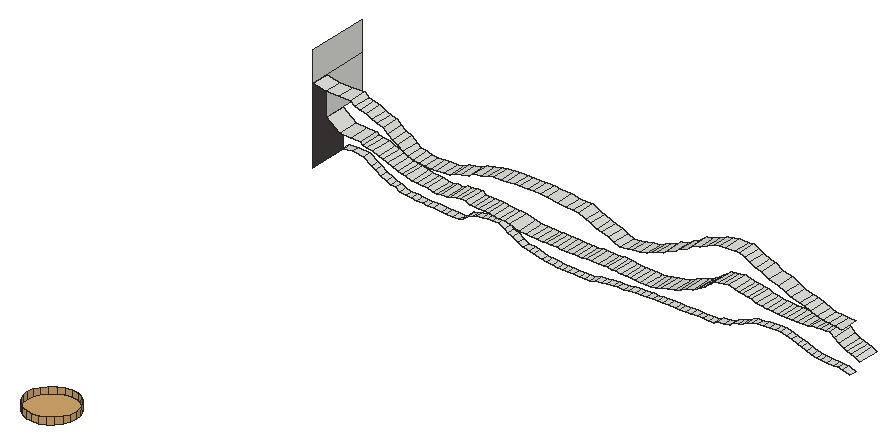
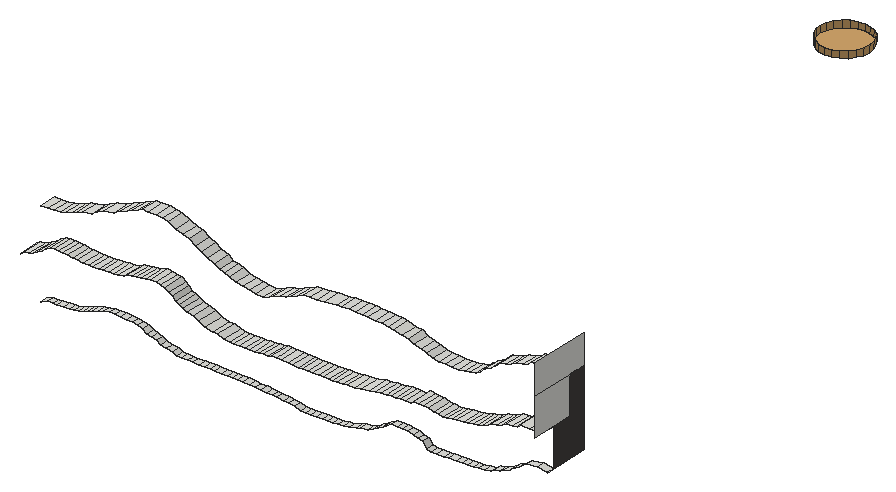
# SketchUp Ruby script. Lengths in inches.
U = 1.inch
M = Sketchup.active_model
def pt(a) = Geom::Point3d.new(a.map { |v| v * U })
def face(e, loops, mat)
  f = e.add_face(loops[0].map { |a| pt(a) })
  loops[1..].each { |l| e.add_face(l.map { |a| pt(a) }).erase! }
  f.material = f.back_material = mat if mat
  f
end
# faces: each face lists its corners as indices into pts; further lists are holes
def faces(e, pts, list, mat = nil) = list.each { |f| face(e, (f[0].is_a?(Array) ? f : [f]).map { |l| l.map { |i| pts[i] } }, mat) }
# xy, xz, yz: faces in a plane at the given z, y or x. An outline is a flat list of corners, or four numbers for a rectangle; further outlines are holes
def ring(l) = l.size == 4 ? [[l[0], l[1]], [l[2], l[1]], [l[2], l[3]], [l[0], l[3]]] : l.each_slice(2).to_a
def flat(e, list, mat, &to3) = list.each { |f| face(e, (f[0].is_a?(Array) ? f : [f]).map { |l| ring(l).map { |u, v| to3.(u, v) } }, mat) }
def xy(e, z, list, mat = nil) = flat(e, list, mat) { |x, y| [x, y, z] }
def xz(e, y, list, mat = nil) = flat(e, list, mat) { |x, z| [x, y, z] }
def yz(e, x, list, mat = nil) = flat(e, list, mat) { |y, z| [x, y, z] }
def lines(e, pts, list) = list.each { |a, b| e.add_line(pt(pts[a]), pt(pts[b])) }
# prism: a flat outline (further loops are holes) pulled along v
def prism(e, loops, v, mat = nil)
  f = face(e, loops, mat); d = Geom::Vector3d.new(v.map { |x| x * U })
  f.pushpull(f.normal.samedirection?(d) ? d.length : -d.length)
end
def box(e, o, s, mat = nil) = prism(e, [[o, [o[0] + s[0], o[1], o[2]], [o[0] + s[0], o[1] + s[1], o[2]], [o[0], o[1] + s[1], o[2]]]], [0, 0, s[2]], mat)
def at(x, y, z, deg = 0) = Geom::Transformation.translation(pt([x, y, z])) * Geom::Transformation.rotation(ORIGIN, Z_AXIS, deg.degrees)
def axes(o, x, y, z) = Geom::Transformation.new([*x, 0, *y, 0, *z, 0, *pt(o).to_a, 1])
def part(name) = M.definitions.add(name)
# library, detail: a bought-in or finely detailed component or shape, given as its bounding box
def library(name, o, s) = part(name).tap { |d| box(d.entities, o, s) }
def detail(e, o, s) = box(e.add_group.entities, o, s)
def put(e, d, t, mat = nil) = e.add_instance(d, t).tap { |i| i.material = mat if mat }
def group(e, t, mat = nil) = e.add_group.tap { |g| g.transformation = t; g.material = mat if mat }.entities
root = M.entities
M.materials.add("[Field Square Tile]").color = [211, 167, 108]
M.materials.add("[Granite Tile]1").color = [68, 65, 63]
xy(root,237.65,[[2039.58,565.74,2040.27,566.68],[2040.27,565.74,2040.89,566.68]])
xy(root,238.33,[[2048.68,565.74,2049.23,566.68],[2049.23,565.74,2049.91,566.68]])
xy(root,238.34,[[2050.59,565.74,2051.52,566.68],[2051.52,565.74,2052.01,566.68],[2052.01,565.74,2052.77,566.68],[2052.77,565.74,2053.4,566.68],[2053.4,565.74,2054.15,566.68],
  [2054.15,565.74,2054.77,566.68],[2054.77,565.74,2055.54,566.68],[2055.54,565.74,2056.16,566.68]])
xy(root,241.52,[[2010.28,561.05,2010.34,566.68]])
xy(root,241.68,[[2040.78,563.18,2041.37,565.74]])
xy(root,241.75,[[2043.13,563.18,2044,565.74],[2044,563.18,2044.62,565.74],[2044.62,563.18,2045.13,565.74]])
xy(root,250.6875,[[2030.6,492.27,2029.81,492.375,2029.07,492.68,2028.43,493.17,2027.95,493.8,2027.64,494.54,2027.54,495.33,2027.64,496.125,2027.95,496.86,2028.43,497.5,2029.07,497.98,2029.81,498.29,2030.6,498.39,2031.39,498.29,2032.13,497.98,2032.76,497.5,2033.25,496.86,2033.56,496.125,2033.66,495.33,2033.56,494.54,2033.25,493.8,2032.76,493.17,2032.13,492.68,2031.39,492.375]],"[Field Square Tile]")
xz(root,561.05,[[2010.28,241.52,2010.34,251.5]])
yz(root,2010.34,[[563.18,246.2,568.68,250.88],[561.05,250.88,568.68,254.5]])
yz(root,2010.34,[[561.05,241.52,565.74,241.52,565.74,246.2,563.18,246.2,563.18,250.88,561.05,250.88]],"[Granite Tile]1")
p = [[2040.89,565.74,237.65],[2040.89,566.68,237.65],[2041.56,566.68,237.89],[2041.56,565.74,237.89],[2036.22,565.74,237.76],[2036.22,566.68,237.76],
  [2036.93,566.68,237.71],[2036.93,565.74,237.71],[2037.54,566.68,237.68],[2037.54,565.74,237.68],[2038.14,566.68,237.67],[2038.14,565.74,237.67],
  [2038.89,566.68,237.66],[2038.89,565.74,237.66],[2039.58,566.68,237.65],[2039.58,565.74,237.65],[2034.87,565.74,237.9],[2034.87,566.68,237.9],
  [2035.53,566.68,237.82],[2035.53,565.74,237.82],[2033.93,565.74,238.21],[2033.93,566.68,238.21],[2042.32,566.68,237.94],[2042.32,565.74,237.94],
  [2042.9375,566.68,237.98],[2042.9375,565.74,237.98],[2043.79,566.68,238.1],[2043.79,565.74,238.1],[2044.34,566.68,238.13],[2044.34,565.74,238.13],
  [2045.1,566.68,238.15],[2045.1,565.74,238.15],[2033.46,565.74,238.31],[2033.46,566.68,238.31],[2045.73,566.68,238.26],[2045.73,565.74,238.26],
  [2032.55,565.74,238.43],[2032.55,566.68,238.43],[2046.48,566.68,238.28],[2046.48,565.74,238.28],[2047.11,566.68,238.3],[2047.11,565.74,238.3],
  [2047.96,566.68,238.32],[2047.96,565.74,238.32],[2048.68,566.68,238.33],[2048.68,565.74,238.33],[2049.91,565.74,238.33],[2049.91,566.68,238.33],
  [2050.59,566.68,238.34],[2050.59,565.74,238.34],[2056.16,565.74,238.34],[2056.16,566.68,238.34],[2056.67,566.68,238.59],[2056.67,565.74,238.59],
  [2031.9,565.74,238.74],[2031.9,566.68,238.74],[2072.19,565.74,238.78],[2072.19,566.68,238.78],[2072.97,566.68,238.43],[2072.97,565.74,238.43],
  [2057.49,566.68,238.72],[2057.49,565.74,238.72],[2031.32,565.74,239.11],[2031.32,566.68,239.11],[2058.18,566.68,238.86],[2058.18,565.74,238.86],
  [2021.53,565.74,238.92],[2021.53,566.68,238.92],[2022.57,566.68,238.82],[2022.57,565.74,238.82],[2023.08,566.68,238.8],[2023.08,565.74,238.8],
  [2023.95,566.68,238.79],[2023.95,565.74,238.79],[2024.69,566.68,238.77],[2024.69,565.74,238.77],[2025.22,566.68,238.9375],[2025.22,565.74,238.9375],
  [2069.47,565.74,238.875],[2069.47,566.68,238.875],[2070.22,566.68,238.83],[2070.22,565.74,238.83],[2070.98,566.68,238.8],[2070.98,565.74,238.8],
  [2071.52,566.68,238.79],[2071.52,565.74,238.79],[2019.44,565.74,238.97],[2019.44,566.68,238.97],[2020.14,566.68,238.94],[2020.14,565.74,238.94],
  [2020.84,566.68,238.93],[2020.84,565.74,238.93],[2025.78,566.68,239.55],[2025.78,565.74,239.55],[2058.69,566.68,239.18],[2058.69,565.74,239.18],
  [2068.32,565.74,239.04],[2068.32,566.68,239.04],[2068.9,566.68,238.94],[2068.9,565.74,238.94],[2018.07,565.74,239.09],[2018.07,566.68,239.09],
  [2018.76,566.68,239.03],[2018.76,565.74,239.03],[2067.66,565.74,239.29],[2067.66,566.68,239.29],[2017.29,565.74,239.19],[2017.29,566.68,239.19],
  [2030.74,565.74,239.38],[2030.74,566.68,239.38],[2016.78,565.74,239.52],[2016.78,566.68,239.52],[2059.28,566.68,239.35],[2059.28,565.74,239.35],
  [2067.08,565.74,239.53],[2067.08,566.68,239.53],[2030.28,565.74,239.71],[2030.28,566.68,239.71],[2059.84,566.68,239.52],[2059.84,565.74,239.52],
  [2016.22,565.74,239.64],[2016.22,566.68,239.64],[2060.39,566.68,239.85],[2060.39,565.74,239.85],[2066.55,565.74,239.7],[2066.55,566.68,239.7],
  [2015.77,565.74,239.86],[2015.77,566.68,239.86],[2026.36,566.68,239.69],[2026.36,565.74,239.69],[2026.91,566.68,239.88],[2026.91,565.74,239.88],
  [2029.58,565.74,240.11],[2029.58,566.68,240.11],[2065.86,565.74,239.92],[2065.86,566.68,239.92],[2061.03,566.68,240.03],[2061.03,565.74,240.03],
  [2014.98,565.74,240.2],[2014.98,566.68,240.2],[2027.64,566.68,239.99],[2027.64,565.74,239.99],[2065.23,565.74,240.11],[2065.23,566.68,240.11],
  [2028.23,566.68,240.05],[2028.23,565.74,240.05],[2028.89,566.68,240.09],[2028.89,565.74,240.09],[2061.6875,566.68,240.12],[2061.6875,565.74,240.12],
  [2062.36,566.68,240.19],[2062.36,565.74,240.19],[2064.45,565.74,240.27],[2064.45,566.68,240.27],[2014.38,565.74,240.59],[2014.38,566.68,240.59],
  [2063.125,566.68,240.23],[2063.125,565.74,240.23],[2063.83,566.68,240.25],[2063.83,565.74,240.25],[2013.84,565.74,240.85],[2013.84,566.68,240.85],
  [2012.82,565.74,241.55],[2012.82,566.68,241.55],[2046.76,563.18,241.57],[2046.76,565.74,241.57],[2047.3,565.74,241.53],[2047.3,563.18,241.53],
  [2047.92,565.74,241.51],[2047.92,563.18,241.51],[2048.47,565.74,241.49],[2048.47,563.18,241.49],[2049.17,565.74,241.48],[2049.17,563.18,241.48],
  [2049.83,565.74,241.47],[2049.83,563.18,241.47],[2050.4,565.74,241.46],[2050.4,563.18,241.46],[2051.11,565.74,241.6],[2051.11,563.18,241.6],
  [2010.34,565.74,241.52],[2010.34,566.68,241.52],[2011.55,566.68,241.69],[2011.55,565.74,241.69],[2046.15,563.18,241.66],[2046.15,565.74,241.66],
  [2051.84,565.74,241.85],[2051.84,563.18,241.85],[2037.12,563.18,241.75],[2037.12,565.74,241.75],[2037.57,565.74,241.74],[2037.57,563.18,241.74],
  [2038.12,565.74,241.72],[2038.12,563.18,241.72],[2038.75,565.74,241.71],[2038.75,563.18,241.71],[2039.38,565.74,241.7],[2039.38,563.18,241.7],
  [2040.11,565.74,241.69],[2040.11,563.18,241.69],[2040.78,565.74,241.68],[2040.78,563.18,241.68],[2041.37,563.18,241.68],[2041.37,565.74,241.68],
  [2041.86,565.74,241.67],[2041.86,563.18,241.67],[2042.5625,565.74,241.74],[2042.5625,563.18,241.74],[2043.13,565.74,241.75],[2043.13,563.18,241.75],
  [2045.13,563.18,241.75],[2045.13,565.74,241.75],[2045.62,565.74,241.67],[2045.62,563.18,241.67],[2034.93,563.18,241.89],[2034.93,565.74,241.89],
  [2035.75,565.74,241.83],[2035.75,563.18,241.83],[2036.35,565.74,241.78],[2036.35,563.18,241.78],[2052.51,565.74,241.91],[2052.51,563.18,241.91],
  [2034.16,563.18,241.96],[2034.16,565.74,241.96],[2053.41,565.74,242.1],[2053.41,563.18,242.1],[2032.99,563.18,242.24],[2032.99,565.74,242.24],
  [2054.18,565.74,242.46],[2054.18,563.18,242.46],[2032.32,563.18,242.34],[2032.32,565.74,242.34],[2075.79,563.18,242.51],[2075.79,565.74,242.51],
  [2076.3,565.74,242.21],[2076.3,563.18,242.21],[2031.66,563.18,242.38],[2031.66,565.74,242.38],[2031,563.18,242.48],[2031,565.74,242.48],
  [2022.82,563.18,242.68],[2022.82,565.74,242.68],[2023.49,565.74,242.51],[2023.49,563.18,242.51],[2024.01,565.74,242.46],[2024.01,563.18,242.46],
  [2024.55,565.74,242.58],[2024.55,563.18,242.58],[2030.36,563.18,242.57],[2030.36,565.74,242.57],[2054.88,565.74,242.78],[2054.88,563.18,242.78],
  [2075.2,563.18,242.68],[2075.2,565.74,242.68],[2025.18,565.74,242.57],[2025.18,563.18,242.57],[2025.81,565.74,242.81],[2025.81,563.18,242.81],
  [2027.58,563.18,242.92],[2027.58,565.74,242.92],[2028.01,565.74,242.625],[2028.01,563.18,242.625],[2028.62,565.74,242.65],[2028.62,563.18,242.65],
  [2029.17,565.74,242.62],[2029.17,563.18,242.62],[2029.8,565.74,242.58],[2029.8,563.18,242.58],[2021.47,563.18,242.78],[2021.47,565.74,242.78],
  [2022.28,565.74,242.73],[2022.28,563.18,242.73],[2074.7,563.18,242.875],[2074.7,565.74,242.875],[2020.17,563.18,243.06],[2020.17,565.74,243.06],
  [2020.89,565.74,242.85],[2020.89,563.18,242.85],[2026.38,565.74,242.86],[2026.38,563.18,242.86],[2055.65,565.74,242.97],[2055.65,563.18,242.97],
  [2026.94,565.74,242.89],[2026.94,563.18,242.89],[2074.31,563.18,243.09],[2074.31,565.74,243.09],[2056.18,565.74,243.23],[2056.18,563.18,243.23],
  [2019.1,563.18,243.3],[2019.1,565.74,243.3],[2019.6875,565.74,243.14],[2019.6875,563.18,243.14],[2073.7,563.18,243.43],[2073.7,565.74,243.43],
  [2056.58,565.74,243.48],[2056.58,563.18,243.48],[2018.46,563.18,243.48],[2018.46,565.74,243.48],[2073.16,563.18,243.8],[2073.16,565.74,243.8],
  [2017.94,563.18,243.79],[2017.94,565.74,243.79],[2057.1,565.74,243.72],[2057.1,563.18,243.72],[2057.4375,565.74,244.12],[2057.4375,563.18,244.12],
  [2017.28,563.18,243.95],[2017.28,565.74,243.95],[2072.56,563.18,244.18],[2072.56,565.74,244.18],[2016.76,563.18,244.11],[2016.76,565.74,244.11],
  [2065.38,563.18,243.99],[2065.38,565.74,243.99],[2066.1,565.74,243.95],[2066.1,563.18,243.95],[2066.6,565.74,243.93],[2066.6,563.18,243.93],
  [2067.29,565.74,243.91],[2067.29,563.18,243.91],[2067.86,565.74,243.89],[2067.86,563.18,243.89],[2068.56,565.74,243.88],[2068.56,563.18,243.88],
  [2069.21,565.74,243.94],[2069.21,563.18,243.94],[2069.85,565.74,243.95],[2069.85,563.18,243.95],[2070.41,565.74,244.1],[2070.41,563.18,244.1],
  [2064.2,563.18,244.11],[2064.2,565.74,244.11],[2064.76,565.74,244.04],[2064.76,563.18,244.04],[2016.09,563.18,244.41],[2016.09,565.74,244.41],
  [2057.91,565.74,244.39],[2057.91,563.18,244.39],[2063.45,563.18,244.25],[2063.45,565.74,244.25],[2071.04,565.74,244.13],[2071.04,563.18,244.13],
  [2071.52,565.74,244.15],[2071.52,563.18,244.15],[2072.04,565.74,244.17],[2072.04,563.18,244.17],[2062.99,563.18,244.51],[2062.99,565.74,244.51],
  [2015.33,563.18,244.54],[2015.33,565.74,244.54],[2058.39,565.74,244.73],[2058.39,563.18,244.73],[2014.77,563.18,244.61],[2014.77,565.74,244.61],
  [2061.84,563.18,244.67],[2061.84,565.74,244.67],[2062.45,565.74,244.55],[2062.45,563.18,244.55],[2014.55,563.18,244.92],[2014.55,565.74,244.92],
  [2058.875,565.74,244.87],[2058.875,563.18,244.87],[2060.79,563.18,244.81],[2060.79,565.74,244.81],[2061.36,565.74,244.7],[2061.36,563.18,244.7],
  [2060.14,563.18,245.01],[2060.14,565.74,245.01],[2011.91,563.18,244.96],[2011.91,565.74,244.96],[2013.3,565.74,244.9375],[2013.3,563.18,244.9375],
  [2059.46,565.74,244.95],[2059.46,563.18,244.95],[2010.34,563.18,246.2],[2010.34,565.74,246.2],[2047.59,561.05,246.35],[2047.59,563.18,246.35],
  [2048.36,563.18,246.05],[2048.36,561.05,246.05],[2049.26,563.18,246.13],[2049.26,561.05,246.13],[2049.97,563.18,246.29],[2049.97,561.05,246.29],
  [2050.77,563.18,246.41],[2050.77,561.05,246.41],[2046.98,561.05,246.66],[2046.98,563.18,246.66],[2051.68,563.18,246.55],[2051.68,561.05,246.55],
  [2023.4,561.05,246.62],[2023.4,563.18,246.62],[2024.14,563.18,246.54],[2024.14,561.05,246.54],[2024.92,563.18,246.51],[2024.92,561.05,246.51],
  [2025.7,563.18,246.58],[2025.7,561.05,246.58],[2074.89,561.05,246.59],[2074.89,563.18,246.59],[2075.78,563.18,246.55],[2075.78,561.05,246.55],
  [2022.74,561.05,246.73],[2022.74,563.18,246.73],[2026.5,563.18,246.59],[2026.5,561.05,246.59],[2027.3,563.18,246.69],[2027.3,561.05,246.69],
  [2052.41,563.18,246.92],[2052.41,561.05,246.92],[2074.18,561.05,246.66],[2074.18,563.18,246.66],[2022.02,561.05,246.88],[2022.02,563.18,246.88],
  [2028.01,563.18,247.03],[2028.01,561.05,247.03],[2046.125,561.05,246.94],[2046.125,563.18,246.94],[2073.39,561.05,246.75],[2073.39,563.18,246.75],
  [2072.7,561.05,246.95],[2072.7,563.18,246.95],[2021.47,561.05,247.25],[2021.47,563.18,247.25],[2045.44,561.05,247.08],[2045.44,563.18,247.08],
  [2053.02,563.18,247.12],[2053.02,561.05,247.12],[2028.7,563.18,247.2],[2028.7,561.05,247.2],[2071.89,561.05,247.25],[2071.89,563.18,247.25],
  [2044.76,561.05,247.46],[2044.76,563.18,247.46],[2053.7,563.18,247.31],[2053.7,561.05,247.31],[2029.67,563.18,247.39],[2029.67,561.05,247.39],
  [2071.21,561.05,247.53],[2071.21,563.18,247.53],[2020.83,561.05,247.72],[2020.83,563.18,247.72],[2054.27,563.18,247.71],[2054.27,561.05,247.71],
  [2030.3,563.18,247.78],[2030.3,561.05,247.78],[2044.13,561.05,247.66],[2044.13,563.18,247.66],[2070.63,561.05,247.66],[2070.63,563.18,247.66],
  [2020.18,561.05,248.07],[2020.18,563.18,248.07],[2043.29,561.05,248.08],[2043.29,563.18,248.08],[2055.2,563.18,248.03],[2055.2,561.05,248.03],
  [2069.5,561.05,247.9],[2069.5,563.18,247.9],[2031.08,563.18,247.89],[2031.08,561.05,247.89],[2032.08,563.18,248.18],[2032.08,561.05,248.18],
  [2068.9,561.05,248.26],[2068.9,563.18,248.26],[2055.91,563.18,248.46],[2055.91,561.05,248.46],[2019.55,561.05,248.51],[2019.55,563.18,248.51],
  [2041.67,561.05,248.15],[2041.67,563.18,248.15],[2042.49,563.18,248.11],[2042.49,561.05,248.11],[2032.72,563.18,248.29],[2032.72,561.05,248.29],
  [2040.64,561.05,248.28],[2040.64,563.18,248.28],[2033.61,563.18,248.35],[2033.61,561.05,248.35],[2039.24,561.05,248.39],[2039.24,563.18,248.39],
  [2067.99,561.05,248.69],[2067.99,563.18,248.69],[2034.34,563.18,248.4],[2034.34,561.05,248.4],[2035.33,563.18,248.4375],[2035.33,561.05,248.4375],
  [2035.99,563.18,248.46],[2035.99,561.05,248.46],[2038.51,561.05,248.49],[2038.51,563.18,248.49],[2019.06,561.05,249.01],[2019.06,563.18,249.01],
  [2036.88,563.18,248.47],[2036.88,561.05,248.47],[2037.62,563.18,248.48],[2037.62,561.05,248.48],[2056.69,563.18,248.82],[2056.69,561.05,248.82],
  [2066.77,561.05,248.95],[2066.77,563.18,248.95],[2057.41,563.18,249.37],[2057.41,561.05,249.37],[2065.88,561.05,249.46],[2065.88,563.18,249.46],
  [2018.29,561.05,249.2],[2018.29,563.18,249.2],[2017.62,561.05,249.41],[2017.62,563.18,249.41],[2016.95,561.05,249.8],[2016.95,563.18,249.8],
  [2058.2,563.18,249.5625],[2058.2,561.05,249.5625],[2065.12,561.05,249.68],[2065.12,563.18,249.68],[2059.1,563.18,249.9],[2059.1,561.05,249.9],
  [2064.46,561.05,250.0625],[2064.46,563.18,250.0625],[2016.15,561.05,249.97],[2016.15,563.18,249.97],[2060.02,563.18,250.35],[2060.02,561.05,250.35],
  [2015.54,561.05,250.15],[2015.54,563.18,250.15],[2015.01,561.05,250.55],[2015.01,563.18,250.55],[2063.77,561.05,250.32],[2063.77,563.18,250.32],
  [2060.68,563.18,250.49],[2060.68,561.05,250.49],[2063.15,561.05,250.61],[2063.15,563.18,250.61],[2010.34,561.05,250.88],[2010.34,563.18,250.88],
  [2011.93,563.18,250.53],[2011.93,561.05,250.53],[2013.55,563.18,250.54],[2013.55,561.05,250.54],[2061.49,563.18,250.6],[2061.49,561.05,250.6],
  [2062.51,563.18,250.58],[2062.51,561.05,250.58],[2030.6,492.27,251.5],[2029.81,492.375,251.5],[2029.81,492.375,250.6875],[2030.6,492.27,250.6875],
  [2031.39,492.375,251.5],[2031.39,492.375,250.6875],[2029.07,492.68,251.5],[2029.07,492.68,250.6875],[2032.13,492.68,251.5],[2032.13,492.68,250.6875],
  [2028.43,493.17,251.5],[2028.43,493.17,250.6875],[2032.76,493.17,251.5],[2032.76,493.17,250.6875],[2027.95,493.8,251.5],[2027.95,493.8,250.6875],
  [2033.25,493.8,251.5],[2033.25,493.8,250.6875],[2027.64,494.54,251.5],[2027.64,494.54,250.6875],[2033.56,494.54,251.5],[2033.56,494.54,250.6875],
  [2027.54,495.33,251.5],[2027.54,495.33,250.6875],[2033.66,495.33,251.5],[2033.66,495.33,250.6875],[2027.64,496.125,251.5],[2027.64,496.125,250.6875],
  [2033.56,496.125,251.5],[2033.56,496.125,250.6875],[2027.95,496.86,251.5],[2027.95,496.86,250.6875],[2033.25,496.86,251.5],[2033.25,496.86,250.6875],
  [2028.43,497.5,251.5],[2028.43,497.5,250.6875],[2032.76,497.5,251.5],[2032.76,497.5,250.6875],[2029.07,497.98,251.5],[2029.07,497.98,250.6875],
  [2032.13,497.98,251.5],[2032.13,497.98,250.6875],[2029.81,498.29,251.5],[2029.81,498.29,250.6875],[2031.39,498.29,251.5],[2031.39,498.29,250.6875],
  [2030.6,498.39,251.5],[2030.6,498.39,250.6875]]
faces(root,p,[[0,1,2,3],[4,5,6,7],[7,6,8,9],[9,8,10,11],[11,10,12,13],[13,12,14,15],[16,17,18,19],[19,18,5,4],
  [20,21,17,16],[3,2,22,23],[23,22,24,25],[25,24,26,27],[27,26,28,29],[29,28,30,31],[32,33,21,20],[31,30,34,35],
  [36,37,33,32],[35,34,38,39],[39,38,40,41],[41,40,42,43],[43,42,44,45],[46,47,48,49],[50,51,52,53],[54,55,37,36],
  [56,57,58,59],[53,52,60,61],[62,63,55,54],[61,60,64,65],[66,67,68,69],[69,68,70,71],[71,70,72,73],[73,72,74,75],
  [75,74,76,77],[78,79,80,81],[81,80,82,83],[83,82,84,85],[85,84,57,56],[86,87,88,89],[89,88,90,91],[91,90,67,66],
  [77,76,92,93],[65,64,94,95],[96,97,98,99],[99,98,79,78],[100,101,102,103],[103,102,87,86],[104,105,97,96],[106,107,101,100],
  [108,109,63,62],[110,111,107,106],[95,94,112,113],[114,115,105,104],[116,117,109,108],[113,112,118,119],[120,121,111,110],[119,118,122,123],
  [124,125,115,114],[126,127,121,120],[93,92,128,129],[129,128,130,131],[132,133,117,116],[134,135,125,124],[123,122,136,137],[138,139,127,126],
  [131,130,140,141],[142,143,135,134],[141,140,144,145],[145,144,146,147],[137,136,148,149],[147,146,133,132],[149,148,150,151],[152,153,143,142],
  [154,155,139,138],[151,150,156,157],[157,156,158,159],[159,158,153,152],[160,161,155,154],[162,163,161,160],[164,165,166,167],[167,166,168,169],
  [169,168,170,171],[171,170,172,173],[173,172,174,175],[175,174,176,177],[177,176,178,179],[180,181,182,183],[184,185,165,164],[179,178,186,187],
  [183,182,163,162],[188,189,190,191],[191,190,192,193],[193,192,194,195],[195,194,196,197],[197,196,198,199],[199,198,200,201],[202,203,204,205],
  [205,204,206,207],[207,206,208,209],[210,211,212,213],[213,212,185,184],[214,215,216,217],[217,216,218,219],[219,218,189,188],[187,186,220,221],
  [222,223,215,214],[221,220,224,225],[226,227,223,222],[225,224,228,229],[230,231,227,226],[232,233,234,235],[236,237,231,230],[238,239,237,236],
  [240,241,242,243],[243,242,244,245],[245,244,246,247],[248,249,239,238],[229,228,250,251],[252,253,233,232],[247,246,254,255],[255,254,256,257],
  [258,259,260,261],[261,260,262,263],[263,262,264,265],[265,264,266,267],[267,266,249,248],[268,269,270,271],[271,270,241,240],[272,273,253,252],
  [274,275,276,277],[277,276,269,268],[257,256,278,279],[251,250,280,281],[279,278,282,283],[283,282,259,258],[284,285,273,272],[281,280,286,287],
  [288,289,290,291],[291,290,275,274],[292,293,285,284],[287,286,294,295],[296,297,289,288],[298,299,293,292],[300,301,297,296],[295,294,302,303],
  [303,302,304,305],[306,307,301,300],[308,309,299,298],[310,311,307,306],[312,313,314,315],[315,314,316,317],[317,316,318,319],[319,318,320,321],
  [321,320,322,323],[323,322,324,325],[325,324,326,327],[327,326,328,329],[330,331,332,333],[333,332,313,312],[334,335,311,310],[305,304,336,337],
  [338,339,331,330],[329,328,340,341],[341,340,342,343],[343,342,344,345],[345,344,309,308],[346,347,339,338],[348,349,335,334],[337,336,350,351],
  [352,353,349,348],[354,355,356,357],[357,356,347,346],[358,359,353,352],[351,350,360,361],[362,363,364,365],[365,364,355,354],[366,367,363,362],
  [368,369,370,371],[371,370,359,358],[361,360,372,373],[373,372,367,366],[374,375,369,368],[376,377,378,379],[379,378,380,381],[381,380,382,383],
  [383,382,384,385],[386,387,377,376],[385,384,388,389],[390,391,392,393],[393,392,394,395],[395,394,396,397],[398,399,400,401],[402,403,391,390],
  [397,396,404,405],[405,404,406,407],[389,388,408,409],[410,411,399,398],[412,413,403,402],[407,406,414,415],[416,417,387,386],[418,419,411,410],
  [420,421,419,418],[422,423,413,412],[424,425,417,416],[409,408,426,427],[415,414,428,429],[430,431,421,420],[432,433,425,424],[427,426,434,435],
  [429,428,436,437],[438,439,431,430],[440,441,423,422],[435,434,442,443],[437,436,444,445],[446,447,433,432],[448,449,439,438],[450,451,441,440],
  [452,453,447,446],[443,442,454,455],[456,457,449,448],[445,444,458,459],[459,458,460,461],[462,463,457,456],[455,454,464,465],[466,467,451,450],
  [468,469,470,471],[471,470,453,452],[461,460,472,473],[474,475,469,468],[473,472,476,477],[478,479,475,474],[480,481,463,462],[477,476,482,483],
  [483,482,484,485],[485,484,486,487],[488,489,479,478],[490,491,467,466],[487,486,492,493],[493,492,494,495],[495,494,489,488],[465,464,496,497],
  [498,499,481,480],[497,496,500,501],[502,503,499,498],[504,505,491,490],[506,507,505,504],[508,509,507,506],[501,500,510,511],[512,513,503,502],
  [511,510,514,515],[516,517,513,512],[518,519,509,508],[515,514,520,521],[522,523,519,518],[524,525,523,522],[526,527,517,516],[521,520,528,529],
  [530,531,527,526],[532,533,534,535],[535,534,536,537],[537,536,525,524],[529,528,538,539],[539,538,540,541],[541,540,531,530]])
faces(root,p,[[542,543,544,545],[546,542,545,547],[543,548,549,544],[550,546,547,551],[548,552,553,549],[554,550,551,555],[552,556,557,553],[558,554,555,559],
  [556,560,561,557],[562,558,559,563],[560,564,565,561],[566,562,563,567],[564,568,569,565],[570,566,567,571],[568,572,573,569],[574,570,571,575],
  [572,576,577,573],[578,574,575,579],[576,580,581,577],[582,578,579,583],[580,584,585,581],[586,582,583,587],[584,588,589,585],[588,586,587,589]],"[Field Square Tile]")
